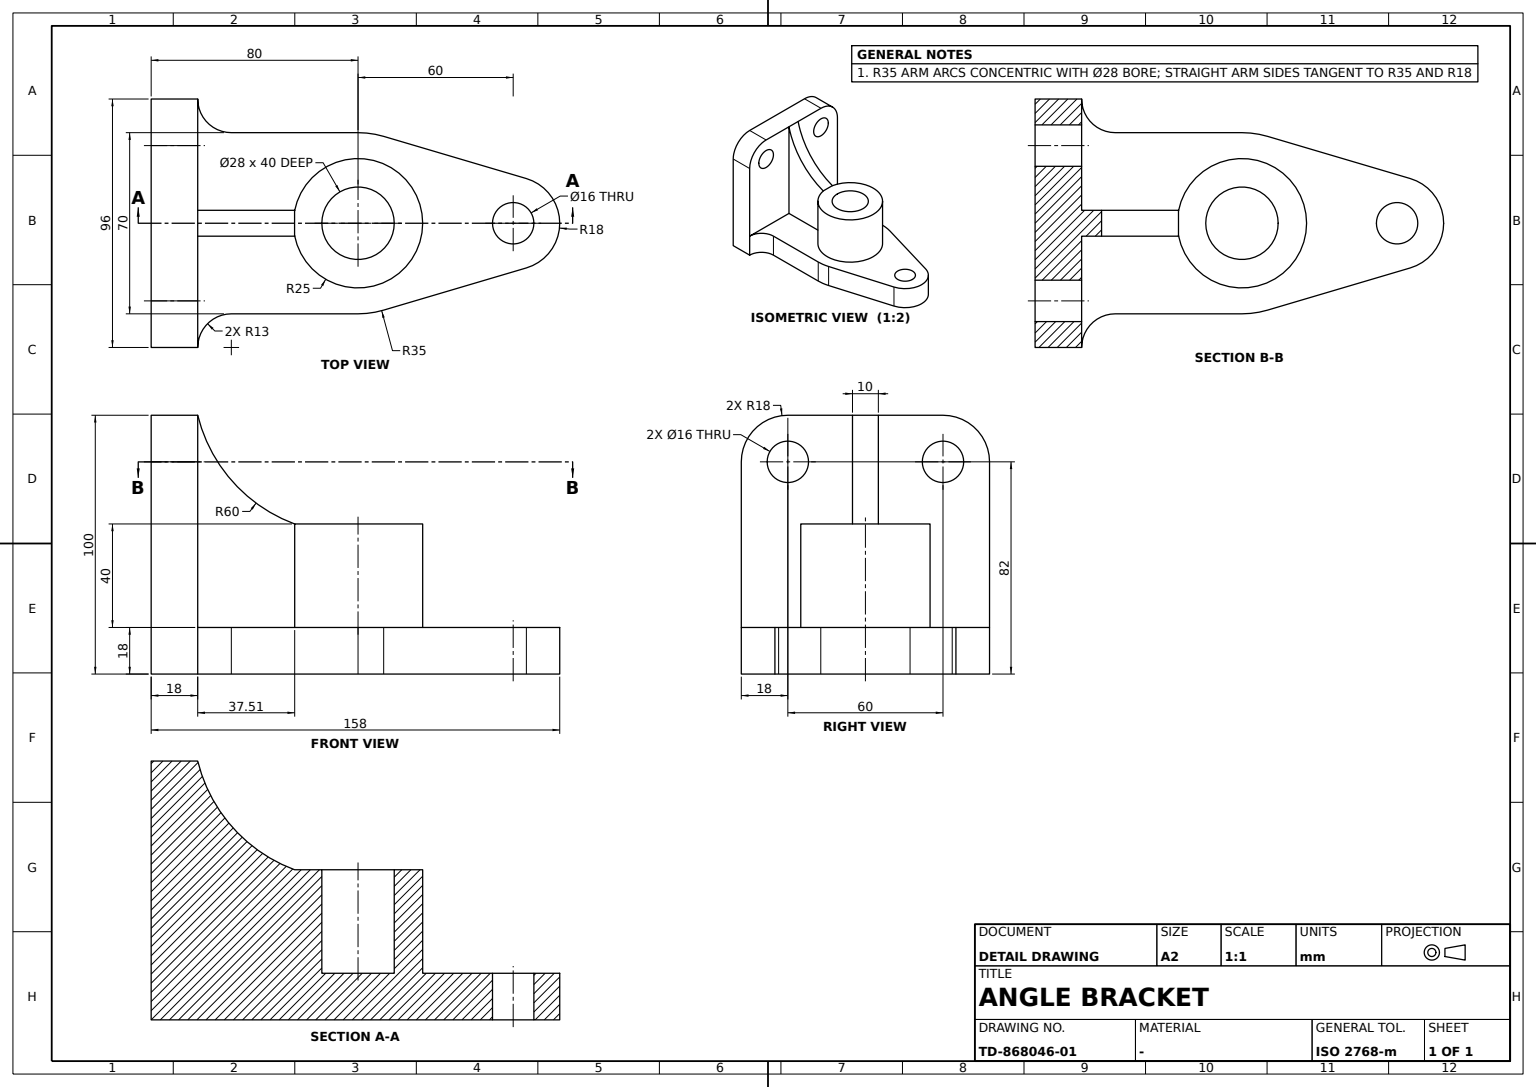
ISO-10303-21;
HEADER;
FILE_DESCRIPTION((''),'2;1');
FILE_NAME('','',(''),(''),'','','');
FILE_SCHEMA(('AUTOMOTIVE_DESIGN'));
ENDSEC;
DATA;
#1=APPLICATION_CONTEXT('');
#2=PRODUCT_CONTEXT('',#1,'mechanical');
#3=PRODUCT('','','',(#2));
#4=PRODUCT_DEFINITION_FORMATION('','',#3);
#5=PRODUCT_DEFINITION_CONTEXT('',#1,'design');
#6=PRODUCT_DEFINITION('','',#4,#5);
#7=PRODUCT_DEFINITION_SHAPE('','',#6);
#8=(LENGTH_UNIT()NAMED_UNIT(*)SI_UNIT(.MILLI.,.METRE.));
#9=(NAMED_UNIT(*)PLANE_ANGLE_UNIT()SI_UNIT($,.RADIAN.));
#10=(NAMED_UNIT(*)SI_UNIT($,.STERADIAN.)SOLID_ANGLE_UNIT());
#11=UNCERTAINTY_MEASURE_WITH_UNIT(LENGTH_MEASURE(1.E-05),#8,'distance_accuracy_value','');
#12=(GEOMETRIC_REPRESENTATION_CONTEXT(3)GLOBAL_UNCERTAINTY_ASSIGNED_CONTEXT((#11))GLOBAL_UNIT_ASSIGNED_CONTEXT((#8,#9,#10))REPRESENTATION_CONTEXT('',''));
#13=CARTESIAN_POINT('',(18.,5.,18.));
#14=VERTEX_POINT('',#13);
#15=CARTESIAN_POINT('',(55.505103,5.,18.));
#16=VERTEX_POINT('',#15);
#17=CARTESIAN_POINT('',(36.752551,5.,18.));
#18=DIRECTION('',(1.,0.,0.));
#19=VECTOR('',#18,1000.);
#20=LINE('',#17,#19);
#21=EDGE_CURVE('',#14,#16,#20,.T.);
#22=ORIENTED_EDGE('',*,*,#21,.F.);
#23=CARTESIAN_POINT('',(18.,5.,100.));
#24=VERTEX_POINT('',#23);
#25=CARTESIAN_POINT('',(18.,5.,59.));
#26=DIRECTION('',(0.,0.,-1.));
#27=VECTOR('',#26,1000.);
#28=LINE('',#25,#27);
#29=EDGE_CURVE('',#24,#14,#28,.T.);
#30=ORIENTED_EDGE('',*,*,#29,.F.);
#31=CARTESIAN_POINT('',(55.458542,5.,58.));
#32=VERTEX_POINT('',#31);
#33=CARTESIAN_POINT('',(76.277827,5.,114.272172));
#34=DIRECTION('',(0.,1.,0.));
#35=DIRECTION('',(-1.,0.,0.));
#36=AXIS2_PLACEMENT_3D('',#33,#34,#35);
#37=CIRCLE('',#36,60.);
#38=EDGE_CURVE('',#32,#24,#37,.T.);
#39=ORIENTED_EDGE('',*,*,#38,.F.);
#40=CARTESIAN_POINT('',(55.505103,5.,57.982774));
#41=VERTEX_POINT('',#40);
#42=CARTESIAN_POINT('',(55.481822,5.,57.991387));
#43=DIRECTION('',(-0.937869538,0.,0.346988082));
#44=VECTOR('',#43,1000.);
#45=LINE('',#42,#44);
#46=EDGE_CURVE('',#41,#32,#45,.T.);
#47=ORIENTED_EDGE('',*,*,#46,.F.);
#48=CARTESIAN_POINT('',(55.505103,5.,37.991387));
#49=DIRECTION('',(0.,0.,1.));
#50=VECTOR('',#49,1000.);
#51=LINE('',#48,#50);
#52=EDGE_CURVE('',#16,#41,#51,.T.);
#53=ORIENTED_EDGE('',*,*,#52,.F.);
#54=EDGE_LOOP('',(#22,#30,#39,#47,#53));
#55=FACE_OUTER_BOUND('',#54,.T.);
#56=CARTESIAN_POINT('',(0.,5.,0.));
#57=AXIS2_PLACEMENT_3D('',#56,#34,#35);
#58=PLANE('',#57);
#59=ADVANCED_FACE('',(#55),#58,.T.);
#60=CARTESIAN_POINT('',(18.,48.,18.));
#61=VERTEX_POINT('',#60);
#62=CARTESIAN_POINT('',(18.,26.5,18.));
#63=VECTOR('',#34,1000.);
#64=LINE('',#62,#63);
#65=EDGE_CURVE('',#14,#61,#64,.T.);
#66=ORIENTED_EDGE('',*,*,#65,.T.);
#67=CARTESIAN_POINT('',(18.,48.,82.));
#68=VERTEX_POINT('',#67);
#69=CARTESIAN_POINT('',(18.,48.,50.));
#70=LINE('',#69,#27);
#71=EDGE_CURVE('',#68,#61,#70,.T.);
#72=ORIENTED_EDGE('',*,*,#71,.F.);
#73=CARTESIAN_POINT('',(18.,30.,100.));
#74=VERTEX_POINT('',#73);
#75=CARTESIAN_POINT('',(18.,30.,82.));
#76=AXIS2_PLACEMENT_3D('',#75,#35,#26);
#77=CIRCLE('',#76,18.);
#78=EDGE_CURVE('',#74,#68,#77,.T.);
#79=ORIENTED_EDGE('',*,*,#78,.F.);
#80=CARTESIAN_POINT('',(18.,17.5,100.));
#81=LINE('',#80,#63);
#82=EDGE_CURVE('',#24,#74,#81,.T.);
#83=ORIENTED_EDGE('',*,*,#82,.F.);
#84=ORIENTED_EDGE('',*,*,#29,.T.);
#85=EDGE_LOOP('',(#66,#72,#79,#83,#84));
#86=FACE_OUTER_BOUND('',#85,.T.);
#87=CARTESIAN_POINT('',(18.,22.,82.));
#88=VERTEX_POINT('',#87);
#89=CARTESIAN_POINT('',(18.,38.,82.));
#90=VERTEX_POINT('',#89);
#91=AXIS2_PLACEMENT_3D('',#75,#18,#34);
#92=CIRCLE('',#91,8.);
#93=EDGE_CURVE('',#88,#90,#92,.T.);
#94=ORIENTED_EDGE('',*,*,#93,.F.);
#95=EDGE_CURVE('',#90,#88,#92,.T.);
#96=ORIENTED_EDGE('',*,*,#95,.F.);
#97=EDGE_LOOP('',(#94,#96));
#98=FACE_BOUND('',#97,.T.);
#99=CARTESIAN_POINT('',(18.,0.,100.));
#100=AXIS2_PLACEMENT_3D('',#99,#18,#26);
#101=PLANE('',#100);
#102=ADVANCED_FACE('',(#86,#98),#101,.T.);
#103=CARTESIAN_POINT('',(0.,-22.,82.));
#104=VERTEX_POINT('',#103);
#105=CARTESIAN_POINT('',(0.,-38.,82.));
#106=VERTEX_POINT('',#105);
#107=CARTESIAN_POINT('',(0.,-30.,82.));
#108=AXIS2_PLACEMENT_3D('',#107,#35,#49);
#109=CIRCLE('',#108,8.);
#110=EDGE_CURVE('',#104,#106,#109,.T.);
#111=ORIENTED_EDGE('',*,*,#110,.T.);
#112=CARTESIAN_POINT('',(18.,-38.,82.));
#113=VERTEX_POINT('',#112);
#114=CARTESIAN_POINT('',(-6.,-38.,82.));
#115=VECTOR('',#35,1000.);
#116=LINE('',#114,#115);
#117=EDGE_CURVE('',#113,#106,#116,.T.);
#118=ORIENTED_EDGE('',*,*,#117,.F.);
#119=CARTESIAN_POINT('',(18.,-22.,82.));
#120=VERTEX_POINT('',#119);
#121=CARTESIAN_POINT('',(18.,-30.,82.));
#122=AXIS2_PLACEMENT_3D('',#121,#18,#34);
#123=CIRCLE('',#122,8.);
#124=EDGE_CURVE('',#113,#120,#123,.T.);
#125=ORIENTED_EDGE('',*,*,#124,.T.);
#126=CARTESIAN_POINT('',(-6.,-22.,82.));
#127=LINE('',#126,#115);
#128=EDGE_CURVE('',#120,#104,#127,.T.);
#129=ORIENTED_EDGE('',*,*,#128,.T.);
#130=EDGE_LOOP('',(#111,#118,#125,#129));
#131=FACE_OUTER_BOUND('',#130,.T.);
#132=CARTESIAN_POINT('',(-6.,-30.,82.));
#133=AXIS2_PLACEMENT_3D('',#132,#35,#34);
#134=CYLINDRICAL_SURFACE('',#133,8.);
#135=ADVANCED_FACE('',(#131),#134,.F.);
#136=CARTESIAN_POINT('',(0.,22.,82.));
#137=VERTEX_POINT('',#136);
#138=CARTESIAN_POINT('',(-6.,22.,82.));
#139=LINE('',#138,#115);
#140=EDGE_CURVE('',#88,#137,#139,.T.);
#141=ORIENTED_EDGE('',*,*,#140,.T.);
#142=CARTESIAN_POINT('',(0.,38.,82.));
#143=VERTEX_POINT('',#142);
#144=CARTESIAN_POINT('',(0.,30.,82.));
#145=AXIS2_PLACEMENT_3D('',#144,#35,#49);
#146=CIRCLE('',#145,8.);
#147=EDGE_CURVE('',#137,#143,#146,.T.);
#148=ORIENTED_EDGE('',*,*,#147,.T.);
#149=CARTESIAN_POINT('',(-6.,38.,82.));
#150=LINE('',#149,#115);
#151=EDGE_CURVE('',#90,#143,#150,.T.);
#152=ORIENTED_EDGE('',*,*,#151,.F.);
#153=ORIENTED_EDGE('',*,*,#95,.T.);
#154=EDGE_LOOP('',(#141,#148,#152,#153));
#155=FACE_OUTER_BOUND('',#154,.T.);
#156=CARTESIAN_POINT('',(-6.,30.,82.));
#157=AXIS2_PLACEMENT_3D('',#156,#35,#34);
#158=CYLINDRICAL_SURFACE('',#157,8.);
#159=ADVANCED_FACE('',(#155),#158,.F.);
#160=ORIENTED_EDGE('',*,*,#110,.F.);
#161=EDGE_CURVE('',#106,#104,#109,.T.);
#162=ORIENTED_EDGE('',*,*,#161,.F.);
#163=EDGE_LOOP('',(#160,#162));
#164=FACE_BOUND('',#163,.T.);
#165=CARTESIAN_POINT('',(0.,-30.,100.));
#166=VERTEX_POINT('',#165);
#167=CARTESIAN_POINT('',(0.,30.,100.));
#168=VERTEX_POINT('',#167);
#169=CARTESIAN_POINT('',(0.,0.,100.));
#170=LINE('',#169,#63);
#171=EDGE_CURVE('',#166,#168,#170,.T.);
#172=ORIENTED_EDGE('',*,*,#171,.T.);
#173=CARTESIAN_POINT('',(0.,48.,82.));
#174=VERTEX_POINT('',#173);
#175=AXIS2_PLACEMENT_3D('',#144,#18,#49);
#176=CIRCLE('',#175,18.);
#177=EDGE_CURVE('',#174,#168,#176,.T.);
#178=ORIENTED_EDGE('',*,*,#177,.F.);
#179=CARTESIAN_POINT('',(0.,48.,0.));
#180=VERTEX_POINT('',#179);
#181=CARTESIAN_POINT('',(0.,48.,41.));
#182=LINE('',#181,#50);
#183=EDGE_CURVE('',#180,#174,#182,.T.);
#184=ORIENTED_EDGE('',*,*,#183,.F.);
#185=CARTESIAN_POINT('',(0.,-48.,0.));
#186=VERTEX_POINT('',#185);
#187=CARTESIAN_POINT('',(0.,0.,0.));
#188=LINE('',#187,#63);
#189=EDGE_CURVE('',#186,#180,#188,.T.);
#190=ORIENTED_EDGE('',*,*,#189,.F.);
#191=CARTESIAN_POINT('',(0.,-48.,82.));
#192=VERTEX_POINT('',#191);
#193=CARTESIAN_POINT('',(0.,-48.,41.));
#194=LINE('',#193,#50);
#195=EDGE_CURVE('',#186,#192,#194,.T.);
#196=ORIENTED_EDGE('',*,*,#195,.T.);
#197=AXIS2_PLACEMENT_3D('',#107,#18,#49);
#198=CIRCLE('',#197,18.);
#199=EDGE_CURVE('',#166,#192,#198,.T.);
#200=ORIENTED_EDGE('',*,*,#199,.F.);
#201=EDGE_LOOP('',(#172,#178,#184,#190,#196,#200));
#202=FACE_OUTER_BOUND('',#201,.T.);
#203=EDGE_CURVE('',#143,#137,#146,.T.);
#204=ORIENTED_EDGE('',*,*,#203,.F.);
#205=ORIENTED_EDGE('',*,*,#147,.F.);
#206=EDGE_LOOP('',(#204,#205));
#207=FACE_BOUND('',#206,.T.);
#208=AXIS2_PLACEMENT_3D('',#187,#35,#49);
#209=PLANE('',#208);
#210=ADVANCED_FACE('',(#164,#202,#207),#209,.T.);
#211=ORIENTED_EDGE('',*,*,#195,.F.);
#212=CARTESIAN_POINT('',(18.,-48.,0.));
#213=VERTEX_POINT('',#212);
#214=CARTESIAN_POINT('',(9.,-48.,0.));
#215=LINE('',#214,#115);
#216=EDGE_CURVE('',#213,#186,#215,.T.);
#217=ORIENTED_EDGE('',*,*,#216,.F.);
#218=CARTESIAN_POINT('',(18.,-48.,18.));
#219=VERTEX_POINT('',#218);
#220=CARTESIAN_POINT('',(18.,-48.,9.));
#221=LINE('',#220,#50);
#222=EDGE_CURVE('',#213,#219,#221,.T.);
#223=ORIENTED_EDGE('',*,*,#222,.T.);
#224=CARTESIAN_POINT('',(18.,-48.,82.));
#225=VERTEX_POINT('',#224);
#226=CARTESIAN_POINT('',(18.,-48.,50.));
#227=LINE('',#226,#27);
#228=EDGE_CURVE('',#225,#219,#227,.T.);
#229=ORIENTED_EDGE('',*,*,#228,.F.);
#230=CARTESIAN_POINT('',(9.,-48.,82.));
#231=LINE('',#230,#19);
#232=EDGE_CURVE('',#192,#225,#231,.T.);
#233=ORIENTED_EDGE('',*,*,#232,.F.);
#234=EDGE_LOOP('',(#211,#217,#223,#229,#233));
#235=FACE_OUTER_BOUND('',#234,.T.);
#236=AXIS2_PLACEMENT_3D('',#185,#34,#35);
#237=PLANE('',#236);
#238=ADVANCED_FACE('',(#235),#237,.F.);
#239=EDGE_CURVE('',#120,#113,#123,.T.);
#240=ORIENTED_EDGE('',*,*,#239,.F.);
#241=ORIENTED_EDGE('',*,*,#124,.F.);
#242=EDGE_LOOP('',(#240,#241));
#243=FACE_BOUND('',#242,.T.);
#244=CARTESIAN_POINT('',(18.,-5.,100.));
#245=VERTEX_POINT('',#244);
#246=CARTESIAN_POINT('',(18.,-5.,18.));
#247=VERTEX_POINT('',#246);
#248=CARTESIAN_POINT('',(18.,-5.,59.));
#249=LINE('',#248,#27);
#250=EDGE_CURVE('',#245,#247,#249,.T.);
#251=ORIENTED_EDGE('',*,*,#250,.F.);
#252=CARTESIAN_POINT('',(18.,-30.,100.));
#253=VERTEX_POINT('',#252);
#254=CARTESIAN_POINT('',(18.,-17.5,100.));
#255=LINE('',#254,#63);
#256=EDGE_CURVE('',#253,#245,#255,.T.);
#257=ORIENTED_EDGE('',*,*,#256,.F.);
#258=AXIS2_PLACEMENT_3D('',#121,#35,#26);
#259=CIRCLE('',#258,18.);
#260=EDGE_CURVE('',#225,#253,#259,.T.);
#261=ORIENTED_EDGE('',*,*,#260,.F.);
#262=ORIENTED_EDGE('',*,*,#228,.T.);
#263=CARTESIAN_POINT('',(18.,-26.5,18.));
#264=LINE('',#263,#63);
#265=EDGE_CURVE('',#219,#247,#264,.T.);
#266=ORIENTED_EDGE('',*,*,#265,.T.);
#267=EDGE_LOOP('',(#251,#257,#261,#262,#266));
#268=FACE_OUTER_BOUND('',#267,.T.);
#269=ADVANCED_FACE('',(#243,#268),#101,.T.);
#270=CARTESIAN_POINT('',(66.,0.,58.));
#271=VERTEX_POINT('',#270);
#272=CARTESIAN_POINT('',(94.,0.,58.));
#273=VERTEX_POINT('',#272);
#274=CARTESIAN_POINT('',(80.,0.,58.));
#275=AXIS2_PLACEMENT_3D('',#274,#49,#18);
#276=CIRCLE('',#275,14.);
#277=EDGE_CURVE('',#271,#273,#276,.T.);
#278=ORIENTED_EDGE('',*,*,#277,.F.);
#279=EDGE_CURVE('',#273,#271,#276,.T.);
#280=ORIENTED_EDGE('',*,*,#279,.F.);
#281=EDGE_LOOP('',(#278,#280));
#282=FACE_BOUND('',#281,.T.);
#283=CARTESIAN_POINT('',(55.458542,-4.766218,58.));
#284=VERTEX_POINT('',#283);
#285=CARTESIAN_POINT('',(105.,0.,58.));
#286=VERTEX_POINT('',#285);
#287=CIRCLE('',#275,25.);
#288=EDGE_CURVE('',#284,#286,#287,.T.);
#289=ORIENTED_EDGE('',*,*,#288,.T.);
#290=CARTESIAN_POINT('',(55.458542,4.766218,58.));
#291=VERTEX_POINT('',#290);
#292=EDGE_CURVE('',#286,#291,#287,.T.);
#293=ORIENTED_EDGE('',*,*,#292,.T.);
#294=CARTESIAN_POINT('',(55.458542,0.,58.));
#295=LINE('',#294,#63);
#296=EDGE_CURVE('',#284,#291,#295,.T.);
#297=ORIENTED_EDGE('',*,*,#296,.F.);
#298=EDGE_LOOP('',(#289,#293,#297));
#299=FACE_OUTER_BOUND('',#298,.T.);
#300=CARTESIAN_POINT('',(0.,0.,58.));
#301=AXIS2_PLACEMENT_3D('',#300,#49,#18);
#302=PLANE('',#301);
#303=ADVANCED_FACE('',(#282,#299),#302,.T.);
#304=CARTESIAN_POINT('',(55.467632,4.813024,57.996637));
#305=CARTESIAN_POINT('',(55.476833,4.859806,57.993233));
#306=CARTESIAN_POINT('',(55.486146,4.906563,57.989787));
#307=CARTESIAN_POINT('',(55.495569,4.953294,57.986301));
#308=B_SPLINE_CURVE_WITH_KNOTS('',5,(#290,#304,#305,#306,#307,#40),.UNSPECIFIED.,.F.,.F.,(6,6),(0.,0.337990946),.UNSPECIFIED.);
#309=EDGE_CURVE('',#291,#41,#308,.T.);
#310=ORIENTED_EDGE('',*,*,#309,.T.);
#311=ORIENTED_EDGE('',*,*,#46,.T.);
#312=CARTESIAN_POINT('',(55.458542,4.883109,58.));
#313=LINE('',#312,#63);
#314=EDGE_CURVE('',#291,#32,#313,.T.);
#315=ORIENTED_EDGE('',*,*,#314,.F.);
#316=EDGE_LOOP('',(#310,#311,#315));
#317=FACE_OUTER_BOUND('',#316,.T.);
#318=DIRECTION('',(0.346988082,0.,0.937869538));
#319=DIRECTION('',(0.937869538,0.,-0.346988082));
#320=AXIS2_PLACEMENT_3D('',#294,#318,#319);
#321=PLANE('',#320);
#322=ADVANCED_FACE('',(#317),#321,.T.);
#323=CARTESIAN_POINT('',(9.,-30.,100.));
#324=LINE('',#323,#19);
#325=EDGE_CURVE('',#166,#253,#324,.T.);
#326=ORIENTED_EDGE('',*,*,#325,.F.);
#327=ORIENTED_EDGE('',*,*,#199,.T.);
#328=ORIENTED_EDGE('',*,*,#232,.T.);
#329=ORIENTED_EDGE('',*,*,#260,.T.);
#330=EDGE_LOOP('',(#326,#327,#328,#329));
#331=FACE_OUTER_BOUND('',#330,.T.);
#332=CARTESIAN_POINT('',(9.,-30.,82.));
#333=DIRECTION('',(0.,-1.,0.));
#334=AXIS2_PLACEMENT_3D('',#332,#35,#333);
#335=CYLINDRICAL_SURFACE('',#334,18.);
#336=ADVANCED_FACE('',(#331),#335,.T.);
#337=CARTESIAN_POINT('',(105.,0.,18.));
#338=VERTEX_POINT('',#337);
#339=CARTESIAN_POINT('',(105.,0.,38.));
#340=LINE('',#339,#50);
#341=EDGE_CURVE('',#338,#286,#340,.T.);
#342=ORIENTED_EDGE('',*,*,#341,.T.);
#343=ORIENTED_EDGE('',*,*,#288,.F.);
#344=CARTESIAN_POINT('',(55.505103,-5.,57.982774));
#345=VERTEX_POINT('',#344);
#346=CARTESIAN_POINT('',(55.467632,-4.813024,57.996637));
#347=CARTESIAN_POINT('',(55.476833,-4.859806,57.993233));
#348=CARTESIAN_POINT('',(55.486146,-4.906563,57.989787));
#349=CARTESIAN_POINT('',(55.495569,-4.953294,57.986301));
#350=B_SPLINE_CURVE_WITH_KNOTS('',5,(#283,#346,#347,#348,#349,#344),.UNSPECIFIED.,.F.,.F.,(6,6),(0.,0.337990946),.UNSPECIFIED.);
#351=EDGE_CURVE('',#284,#345,#350,.T.);
#352=ORIENTED_EDGE('',*,*,#351,.T.);
#353=CARTESIAN_POINT('',(55.505103,-5.,18.));
#354=VERTEX_POINT('',#353);
#355=CARTESIAN_POINT('',(55.505103,-5.,37.991387));
#356=LINE('',#355,#50);
#357=EDGE_CURVE('',#354,#345,#356,.T.);
#358=ORIENTED_EDGE('',*,*,#357,.F.);
#359=CARTESIAN_POINT('',(80.,0.,18.));
#360=AXIS2_PLACEMENT_3D('',#359,#49,#18);
#361=CIRCLE('',#360,25.);
#362=EDGE_CURVE('',#354,#338,#361,.T.);
#363=ORIENTED_EDGE('',*,*,#362,.T.);
#364=EDGE_LOOP('',(#342,#343,#352,#358,#363));
#365=FACE_OUTER_BOUND('',#364,.T.);
#366=CARTESIAN_POINT('',(80.,0.,38.));
#367=AXIS2_PLACEMENT_3D('',#366,#26,#18);
#368=CYLINDRICAL_SURFACE('',#367,25.);
#369=ADVANCED_FACE('',(#365),#368,.T.);
#370=CARTESIAN_POINT('',(158.,0.,18.));
#371=VERTEX_POINT('',#370);
#372=CARTESIAN_POINT('',(158.,0.,0.));
#373=VERTEX_POINT('',#372);
#374=CARTESIAN_POINT('',(158.,0.,9.));
#375=LINE('',#374,#27);
#376=EDGE_CURVE('',#371,#373,#375,.T.);
#377=ORIENTED_EDGE('',*,*,#376,.F.);
#378=CARTESIAN_POINT('',(145.1,-17.262387,18.));
#379=VERTEX_POINT('',#378);
#380=CARTESIAN_POINT('',(140.,0.,18.));
#381=AXIS2_PLACEMENT_3D('',#380,#49,#18);
#382=CIRCLE('',#381,18.);
#383=EDGE_CURVE('',#379,#371,#382,.T.);
#384=ORIENTED_EDGE('',*,*,#383,.F.);
#385=CARTESIAN_POINT('',(145.1,-17.262387,0.));
#386=VERTEX_POINT('',#385);
#387=CARTESIAN_POINT('',(145.1,-17.262387,9.));
#388=LINE('',#387,#50);
#389=EDGE_CURVE('',#386,#379,#388,.T.);
#390=ORIENTED_EDGE('',*,*,#389,.F.);
#391=CARTESIAN_POINT('',(140.,0.,0.));
#392=AXIS2_PLACEMENT_3D('',#391,#49,#18);
#393=CIRCLE('',#392,18.);
#394=EDGE_CURVE('',#386,#373,#393,.T.);
#395=ORIENTED_EDGE('',*,*,#394,.T.);
#396=EDGE_LOOP('',(#377,#384,#390,#395));
#397=FACE_OUTER_BOUND('',#396,.T.);
#398=CARTESIAN_POINT('',(140.,0.,9.));
#399=AXIS2_PLACEMENT_3D('',#398,#26,#18);
#400=CYLINDRICAL_SURFACE('',#399,18.);
#401=ADVANCED_FACE('',(#397),#400,.T.);
#402=CARTESIAN_POINT('',(80.,-35.,0.));
#403=VERTEX_POINT('',#402);
#404=CARTESIAN_POINT('',(80.,-35.,18.));
#405=VERTEX_POINT('',#404);
#406=CARTESIAN_POINT('',(80.,-35.,9.));
#407=LINE('',#406,#50);
#408=EDGE_CURVE('',#403,#405,#407,.T.);
#409=ORIENTED_EDGE('',*,*,#408,.F.);
#410=CARTESIAN_POINT('',(89.916667,-33.565752,0.));
#411=VERTEX_POINT('',#410);
#412=CARTESIAN_POINT('',(80.,0.,0.));
#413=AXIS2_PLACEMENT_3D('',#412,#49,#18);
#414=CIRCLE('',#413,35.);
#415=EDGE_CURVE('',#403,#411,#414,.T.);
#416=ORIENTED_EDGE('',*,*,#415,.T.);
#417=CARTESIAN_POINT('',(89.916667,-33.565752,18.));
#418=VERTEX_POINT('',#417);
#419=CARTESIAN_POINT('',(89.916667,-33.565752,9.));
#420=LINE('',#419,#50);
#421=EDGE_CURVE('',#411,#418,#420,.T.);
#422=ORIENTED_EDGE('',*,*,#421,.T.);
#423=CIRCLE('',#360,35.);
#424=EDGE_CURVE('',#405,#418,#423,.T.);
#425=ORIENTED_EDGE('',*,*,#424,.F.);
#426=EDGE_LOOP('',(#409,#416,#422,#425));
#427=FACE_OUTER_BOUND('',#426,.T.);
#428=CARTESIAN_POINT('',(80.,0.,9.));
#429=AXIS2_PLACEMENT_3D('',#428,#26,#18);
#430=CYLINDRICAL_SURFACE('',#429,35.);
#431=ADVANCED_FACE('',(#427),#430,.T.);
#432=CARTESIAN_POINT('',(148.,0.,0.));
#433=VERTEX_POINT('',#432);
#434=CARTESIAN_POINT('',(132.,0.,0.));
#435=VERTEX_POINT('',#434);
#436=AXIS2_PLACEMENT_3D('',#391,#26,#35);
#437=CIRCLE('',#436,8.);
#438=EDGE_CURVE('',#433,#435,#437,.T.);
#439=ORIENTED_EDGE('',*,*,#438,.F.);
#440=EDGE_CURVE('',#435,#433,#437,.T.);
#441=ORIENTED_EDGE('',*,*,#440,.F.);
#442=EDGE_LOOP('',(#439,#441));
#443=FACE_BOUND('',#442,.T.);
#444=ORIENTED_EDGE('',*,*,#216,.T.);
#445=ORIENTED_EDGE('',*,*,#189,.T.);
#446=CARTESIAN_POINT('',(18.,48.,0.));
#447=VERTEX_POINT('',#446);
#448=CARTESIAN_POINT('',(9.,48.,0.));
#449=LINE('',#448,#115);
#450=EDGE_CURVE('',#447,#180,#449,.T.);
#451=ORIENTED_EDGE('',*,*,#450,.F.);
#452=CARTESIAN_POINT('',(31.,35.,0.));
#453=VERTEX_POINT('',#452);
#454=CARTESIAN_POINT('',(31.,48.,0.));
#455=AXIS2_PLACEMENT_3D('',#454,#49,#35);
#456=CIRCLE('',#455,13.);
#457=EDGE_CURVE('',#447,#453,#456,.T.);
#458=ORIENTED_EDGE('',*,*,#457,.T.);
#459=CARTESIAN_POINT('',(80.,35.,0.));
#460=VERTEX_POINT('',#459);
#461=CARTESIAN_POINT('',(55.5,35.,0.));
#462=LINE('',#461,#115);
#463=EDGE_CURVE('',#460,#453,#462,.T.);
#464=ORIENTED_EDGE('',*,*,#463,.F.);
#465=CARTESIAN_POINT('',(89.916667,33.565752,0.));
#466=VERTEX_POINT('',#465);
#467=EDGE_CURVE('',#466,#460,#414,.T.);
#468=ORIENTED_EDGE('',*,*,#467,.F.);
#469=CARTESIAN_POINT('',(145.1,17.262387,0.));
#470=VERTEX_POINT('',#469);
#471=CARTESIAN_POINT('',(117.508333,25.41407,0.));
#472=DIRECTION('',(-0.959021492,0.283333333,0.));
#473=VECTOR('',#472,1000.);
#474=LINE('',#471,#473);
#475=EDGE_CURVE('',#470,#466,#474,.T.);
#476=ORIENTED_EDGE('',*,*,#475,.F.);
#477=EDGE_CURVE('',#373,#470,#393,.T.);
#478=ORIENTED_EDGE('',*,*,#477,.F.);
#479=ORIENTED_EDGE('',*,*,#394,.F.);
#480=CARTESIAN_POINT('',(117.508333,-25.41407,0.));
#481=DIRECTION('',(0.959021492,0.283333333,0.));
#482=VECTOR('',#481,1000.);
#483=LINE('',#480,#482);
#484=EDGE_CURVE('',#411,#386,#483,.T.);
#485=ORIENTED_EDGE('',*,*,#484,.F.);
#486=ORIENTED_EDGE('',*,*,#415,.F.);
#487=CARTESIAN_POINT('',(31.,-35.,0.));
#488=VERTEX_POINT('',#487);
#489=CARTESIAN_POINT('',(55.5,-35.,0.));
#490=LINE('',#489,#19);
#491=EDGE_CURVE('',#488,#403,#490,.T.);
#492=ORIENTED_EDGE('',*,*,#491,.F.);
#493=CARTESIAN_POINT('',(31.,-48.,0.));
#494=AXIS2_PLACEMENT_3D('',#493,#49,#35);
#495=CIRCLE('',#494,13.);
#496=EDGE_CURVE('',#488,#213,#495,.T.);
#497=ORIENTED_EDGE('',*,*,#496,.T.);
#498=EDGE_LOOP('',(#444,#445,#451,#458,#464,#468,#476,#478,#479,#485,#486,#492,#497));
#499=FACE_OUTER_BOUND('',#498,.T.);
#500=CARTESIAN_POINT('',(18.,0.,0.));
#501=AXIS2_PLACEMENT_3D('',#500,#26,#35);
#502=PLANE('',#501);
#503=ADVANCED_FACE('',(#443,#499),#502,.T.);
#504=ORIENTED_EDGE('',*,*,#484,.T.);
#505=ORIENTED_EDGE('',*,*,#389,.T.);
#506=CARTESIAN_POINT('',(117.508333,-25.41407,18.));
#507=LINE('',#506,#482);
#508=EDGE_CURVE('',#418,#379,#507,.T.);
#509=ORIENTED_EDGE('',*,*,#508,.F.);
#510=ORIENTED_EDGE('',*,*,#421,.F.);
#511=EDGE_LOOP('',(#504,#505,#509,#510));
#512=FACE_OUTER_BOUND('',#511,.T.);
#513=DIRECTION('',(0.283333333,-0.959021492,0.));
#514=AXIS2_PLACEMENT_3D('',#410,#513,#481);
#515=PLANE('',#514);
#516=ADVANCED_FACE('',(#512),#515,.T.);
#517=EDGE_CURVE('',#338,#16,#361,.T.);
#518=ORIENTED_EDGE('',*,*,#517,.T.);
#519=ORIENTED_EDGE('',*,*,#52,.T.);
#520=ORIENTED_EDGE('',*,*,#309,.F.);
#521=ORIENTED_EDGE('',*,*,#292,.F.);
#522=ORIENTED_EDGE('',*,*,#341,.F.);
#523=EDGE_LOOP('',(#518,#519,#520,#521,#522));
#524=FACE_OUTER_BOUND('',#523,.T.);
#525=ADVANCED_FACE('',(#524),#368,.T.);
#526=ORIENTED_EDGE('',*,*,#140,.F.);
#527=ORIENTED_EDGE('',*,*,#93,.T.);
#528=ORIENTED_EDGE('',*,*,#151,.T.);
#529=ORIENTED_EDGE('',*,*,#203,.T.);
#530=EDGE_LOOP('',(#526,#527,#528,#529));
#531=FACE_OUTER_BOUND('',#530,.T.);
#532=ADVANCED_FACE('',(#531),#158,.F.);
#533=CARTESIAN_POINT('',(31.,-35.,18.));
#534=VERTEX_POINT('',#533);
#535=CARTESIAN_POINT('',(31.,-48.,18.));
#536=AXIS2_PLACEMENT_3D('',#535,#26,#18);
#537=CIRCLE('',#536,13.);
#538=EDGE_CURVE('',#219,#534,#537,.T.);
#539=ORIENTED_EDGE('',*,*,#538,.F.);
#540=ORIENTED_EDGE('',*,*,#222,.F.);
#541=ORIENTED_EDGE('',*,*,#496,.F.);
#542=CARTESIAN_POINT('',(31.,-35.,9.));
#543=LINE('',#542,#50);
#544=EDGE_CURVE('',#488,#534,#543,.T.);
#545=ORIENTED_EDGE('',*,*,#544,.T.);
#546=EDGE_LOOP('',(#539,#540,#541,#545));
#547=FACE_OUTER_BOUND('',#546,.T.);
#548=CARTESIAN_POINT('',(31.,-48.,50.));
#549=AXIS2_PLACEMENT_3D('',#548,#26,#35);
#550=CYLINDRICAL_SURFACE('',#549,13.);
#551=ADVANCED_FACE('',(#547),#550,.F.);
#552=ORIENTED_EDGE('',*,*,#517,.F.);
#553=ORIENTED_EDGE('',*,*,#362,.F.);
#554=CARTESIAN_POINT('',(36.752551,-5.,18.));
#555=LINE('',#554,#19);
#556=EDGE_CURVE('',#247,#354,#555,.T.);
#557=ORIENTED_EDGE('',*,*,#556,.F.);
#558=ORIENTED_EDGE('',*,*,#265,.F.);
#559=ORIENTED_EDGE('',*,*,#538,.T.);
#560=CARTESIAN_POINT('',(55.5,-35.,18.));
#561=LINE('',#560,#19);
#562=EDGE_CURVE('',#534,#405,#561,.T.);
#563=ORIENTED_EDGE('',*,*,#562,.T.);
#564=ORIENTED_EDGE('',*,*,#424,.T.);
#565=ORIENTED_EDGE('',*,*,#508,.T.);
#566=ORIENTED_EDGE('',*,*,#383,.T.);
#567=CARTESIAN_POINT('',(145.1,17.262387,18.));
#568=VERTEX_POINT('',#567);
#569=EDGE_CURVE('',#371,#568,#382,.T.);
#570=ORIENTED_EDGE('',*,*,#569,.T.);
#571=CARTESIAN_POINT('',(89.916667,33.565752,18.));
#572=VERTEX_POINT('',#571);
#573=CARTESIAN_POINT('',(117.508333,25.41407,18.));
#574=LINE('',#573,#473);
#575=EDGE_CURVE('',#568,#572,#574,.T.);
#576=ORIENTED_EDGE('',*,*,#575,.T.);
#577=CARTESIAN_POINT('',(80.,35.,18.));
#578=VERTEX_POINT('',#577);
#579=EDGE_CURVE('',#572,#578,#423,.T.);
#580=ORIENTED_EDGE('',*,*,#579,.T.);
#581=CARTESIAN_POINT('',(31.,35.,18.));
#582=VERTEX_POINT('',#581);
#583=CARTESIAN_POINT('',(55.5,35.,18.));
#584=LINE('',#583,#115);
#585=EDGE_CURVE('',#578,#582,#584,.T.);
#586=ORIENTED_EDGE('',*,*,#585,.T.);
#587=CARTESIAN_POINT('',(31.,48.,18.));
#588=AXIS2_PLACEMENT_3D('',#587,#26,#18);
#589=CIRCLE('',#588,13.);
#590=EDGE_CURVE('',#582,#61,#589,.T.);
#591=ORIENTED_EDGE('',*,*,#590,.T.);
#592=ORIENTED_EDGE('',*,*,#65,.F.);
#593=ORIENTED_EDGE('',*,*,#21,.T.);
#594=EDGE_LOOP('',(#552,#553,#557,#558,#559,#563,#564,#565,#566,#570,#576,#580,#586,#591,#592,#593));
#595=FACE_OUTER_BOUND('',#594,.T.);
#596=CARTESIAN_POINT('',(148.,0.,18.));
#597=VERTEX_POINT('',#596);
#598=CARTESIAN_POINT('',(132.,0.,18.));
#599=VERTEX_POINT('',#598);
#600=CIRCLE('',#381,8.);
#601=EDGE_CURVE('',#597,#599,#600,.T.);
#602=ORIENTED_EDGE('',*,*,#601,.F.);
#603=EDGE_CURVE('',#599,#597,#600,.T.);
#604=ORIENTED_EDGE('',*,*,#603,.F.);
#605=EDGE_LOOP('',(#602,#604));
#606=FACE_BOUND('',#605,.T.);
#607=CARTESIAN_POINT('',(0.,0.,18.));
#608=AXIS2_PLACEMENT_3D('',#607,#49,#18);
#609=PLANE('',#608);
#610=ADVANCED_FACE('',(#595,#606),#609,.T.);
#611=CARTESIAN_POINT('',(80.,35.,9.));
#612=LINE('',#611,#50);
#613=EDGE_CURVE('',#460,#578,#612,.T.);
#614=ORIENTED_EDGE('',*,*,#613,.F.);
#615=ORIENTED_EDGE('',*,*,#463,.T.);
#616=CARTESIAN_POINT('',(31.,35.,9.));
#617=LINE('',#616,#50);
#618=EDGE_CURVE('',#453,#582,#617,.T.);
#619=ORIENTED_EDGE('',*,*,#618,.T.);
#620=ORIENTED_EDGE('',*,*,#585,.F.);
#621=EDGE_LOOP('',(#614,#615,#619,#620));
#622=FACE_OUTER_BOUND('',#621,.T.);
#623=CARTESIAN_POINT('',(18.,35.,0.));
#624=AXIS2_PLACEMENT_3D('',#623,#333,#18);
#625=PLANE('',#624);
#626=ADVANCED_FACE('',(#622),#625,.F.);
#627=ORIENTED_EDGE('',*,*,#128,.F.);
#628=ORIENTED_EDGE('',*,*,#239,.T.);
#629=ORIENTED_EDGE('',*,*,#117,.T.);
#630=ORIENTED_EDGE('',*,*,#161,.T.);
#631=EDGE_LOOP('',(#627,#628,#629,#630));
#632=FACE_OUTER_BOUND('',#631,.T.);
#633=ADVANCED_FACE('',(#632),#134,.F.);
#634=CARTESIAN_POINT('',(94.,0.,18.));
#635=VERTEX_POINT('',#634);
#636=CARTESIAN_POINT('',(66.,0.,18.));
#637=VERTEX_POINT('',#636);
#638=CIRCLE('',#360,14.);
#639=EDGE_CURVE('',#635,#637,#638,.T.);
#640=ORIENTED_EDGE('',*,*,#639,.T.);
#641=EDGE_CURVE('',#637,#635,#638,.T.);
#642=ORIENTED_EDGE('',*,*,#641,.T.);
#643=EDGE_LOOP('',(#640,#642));
#644=FACE_OUTER_BOUND('',#643,.T.);
#645=ADVANCED_FACE('',(#644),#609,.T.);
#646=ORIENTED_EDGE('',*,*,#475,.T.);
#647=CARTESIAN_POINT('',(89.916667,33.565752,9.));
#648=LINE('',#647,#50);
#649=EDGE_CURVE('',#466,#572,#648,.T.);
#650=ORIENTED_EDGE('',*,*,#649,.T.);
#651=ORIENTED_EDGE('',*,*,#575,.F.);
#652=CARTESIAN_POINT('',(145.1,17.262387,9.));
#653=LINE('',#652,#50);
#654=EDGE_CURVE('',#470,#568,#653,.T.);
#655=ORIENTED_EDGE('',*,*,#654,.F.);
#656=EDGE_LOOP('',(#646,#650,#651,#655));
#657=FACE_OUTER_BOUND('',#656,.T.);
#658=DIRECTION('',(-0.283333333,-0.959021492,0.));
#659=DIRECTION('',(0.959021492,-0.283333333,0.));
#660=AXIS2_PLACEMENT_3D('',#465,#658,#659);
#661=PLANE('',#660);
#662=ADVANCED_FACE('',(#657),#661,.F.);
#663=ORIENTED_EDGE('',*,*,#279,.T.);
#664=CARTESIAN_POINT('',(66.,0.,38.));
#665=LINE('',#664,#27);
#666=EDGE_CURVE('',#271,#637,#665,.T.);
#667=ORIENTED_EDGE('',*,*,#666,.T.);
#668=ORIENTED_EDGE('',*,*,#639,.F.);
#669=CARTESIAN_POINT('',(94.,0.,38.));
#670=LINE('',#669,#27);
#671=EDGE_CURVE('',#273,#635,#670,.T.);
#672=ORIENTED_EDGE('',*,*,#671,.F.);
#673=EDGE_LOOP('',(#663,#667,#668,#672));
#674=FACE_OUTER_BOUND('',#673,.T.);
#675=CYLINDRICAL_SURFACE('',#367,14.);
#676=ADVANCED_FACE('',(#674),#675,.F.);
#677=ORIENTED_EDGE('',*,*,#438,.T.);
#678=CARTESIAN_POINT('',(132.,0.,-2.));
#679=LINE('',#678,#27);
#680=EDGE_CURVE('',#599,#435,#679,.T.);
#681=ORIENTED_EDGE('',*,*,#680,.F.);
#682=ORIENTED_EDGE('',*,*,#603,.T.);
#683=CARTESIAN_POINT('',(148.,0.,-2.));
#684=LINE('',#683,#27);
#685=EDGE_CURVE('',#597,#433,#684,.T.);
#686=ORIENTED_EDGE('',*,*,#685,.T.);
#687=EDGE_LOOP('',(#677,#681,#682,#686));
#688=FACE_OUTER_BOUND('',#687,.T.);
#689=CARTESIAN_POINT('',(140.,0.,-2.));
#690=AXIS2_PLACEMENT_3D('',#689,#26,#18);
#691=CYLINDRICAL_SURFACE('',#690,8.);
#692=ADVANCED_FACE('',(#688),#691,.F.);
#693=ORIENTED_EDGE('',*,*,#376,.T.);
#694=ORIENTED_EDGE('',*,*,#477,.T.);
#695=ORIENTED_EDGE('',*,*,#654,.T.);
#696=ORIENTED_EDGE('',*,*,#569,.F.);
#697=EDGE_LOOP('',(#693,#694,#695,#696));
#698=FACE_OUTER_BOUND('',#697,.T.);
#699=ADVANCED_FACE('',(#698),#400,.T.);
#700=ORIENTED_EDGE('',*,*,#601,.T.);
#701=ORIENTED_EDGE('',*,*,#680,.T.);
#702=ORIENTED_EDGE('',*,*,#440,.T.);
#703=ORIENTED_EDGE('',*,*,#685,.F.);
#704=EDGE_LOOP('',(#700,#701,#702,#703));
#705=FACE_OUTER_BOUND('',#704,.T.);
#706=ADVANCED_FACE('',(#705),#691,.F.);
#707=CARTESIAN_POINT('',(55.458542,-5.,58.));
#708=VERTEX_POINT('',#707);
#709=CARTESIAN_POINT('',(55.458542,-4.883109,58.));
#710=LINE('',#709,#63);
#711=EDGE_CURVE('',#708,#284,#710,.T.);
#712=ORIENTED_EDGE('',*,*,#711,.F.);
#713=CARTESIAN_POINT('',(55.481822,-5.,57.991387));
#714=LINE('',#713,#44);
#715=EDGE_CURVE('',#345,#708,#714,.T.);
#716=ORIENTED_EDGE('',*,*,#715,.F.);
#717=ORIENTED_EDGE('',*,*,#351,.F.);
#718=EDGE_LOOP('',(#712,#716,#717));
#719=FACE_OUTER_BOUND('',#718,.T.);
#720=ADVANCED_FACE('',(#719),#321,.T.);
#721=CARTESIAN_POINT('',(9.,30.,100.));
#722=LINE('',#721,#19);
#723=EDGE_CURVE('',#168,#74,#722,.T.);
#724=ORIENTED_EDGE('',*,*,#723,.T.);
#725=ORIENTED_EDGE('',*,*,#78,.T.);
#726=CARTESIAN_POINT('',(9.,48.,82.));
#727=LINE('',#726,#19);
#728=EDGE_CURVE('',#174,#68,#727,.T.);
#729=ORIENTED_EDGE('',*,*,#728,.F.);
#730=ORIENTED_EDGE('',*,*,#177,.T.);
#731=EDGE_LOOP('',(#724,#725,#729,#730));
#732=FACE_OUTER_BOUND('',#731,.T.);
#733=CARTESIAN_POINT('',(9.,30.,82.));
#734=AXIS2_PLACEMENT_3D('',#733,#35,#49);
#735=CYLINDRICAL_SURFACE('',#734,18.);
#736=ADVANCED_FACE('',(#732),#735,.T.);
#737=CARTESIAN_POINT('',(76.277827,-5.,114.272172));
#738=AXIS2_PLACEMENT_3D('',#737,#34,#35);
#739=CIRCLE('',#738,60.);
#740=EDGE_CURVE('',#708,#245,#739,.T.);
#741=ORIENTED_EDGE('',*,*,#740,.T.);
#742=ORIENTED_EDGE('',*,*,#250,.T.);
#743=ORIENTED_EDGE('',*,*,#556,.T.);
#744=ORIENTED_EDGE('',*,*,#357,.T.);
#745=ORIENTED_EDGE('',*,*,#715,.T.);
#746=EDGE_LOOP('',(#741,#742,#743,#744,#745));
#747=FACE_OUTER_BOUND('',#746,.T.);
#748=CARTESIAN_POINT('',(0.,-5.,0.));
#749=AXIS2_PLACEMENT_3D('',#748,#34,#35);
#750=PLANE('',#749);
#751=ADVANCED_FACE('',(#747),#750,.F.);
#752=ORIENTED_EDGE('',*,*,#562,.F.);
#753=ORIENTED_EDGE('',*,*,#544,.F.);
#754=ORIENTED_EDGE('',*,*,#491,.T.);
#755=ORIENTED_EDGE('',*,*,#408,.T.);
#756=EDGE_LOOP('',(#752,#753,#754,#755));
#757=FACE_OUTER_BOUND('',#756,.T.);
#758=CARTESIAN_POINT('',(18.,-35.,0.));
#759=AXIS2_PLACEMENT_3D('',#758,#333,#18);
#760=PLANE('',#759);
#761=ADVANCED_FACE('',(#757),#760,.T.);
#762=LINE('',#99,#63);
#763=EDGE_CURVE('',#245,#24,#762,.T.);
#764=ORIENTED_EDGE('',*,*,#763,.T.);
#765=ORIENTED_EDGE('',*,*,#82,.T.);
#766=ORIENTED_EDGE('',*,*,#723,.F.);
#767=ORIENTED_EDGE('',*,*,#171,.F.);
#768=ORIENTED_EDGE('',*,*,#325,.T.);
#769=ORIENTED_EDGE('',*,*,#256,.T.);
#770=EDGE_LOOP('',(#764,#765,#766,#767,#768,#769));
#771=FACE_OUTER_BOUND('',#770,.T.);
#772=AXIS2_PLACEMENT_3D('',#169,#49,#18);
#773=PLANE('',#772);
#774=ADVANCED_FACE('',(#771),#773,.T.);
#775=ORIENTED_EDGE('',*,*,#763,.F.);
#776=ORIENTED_EDGE('',*,*,#740,.F.);
#777=ORIENTED_EDGE('',*,*,#711,.T.);
#778=ORIENTED_EDGE('',*,*,#296,.T.);
#779=ORIENTED_EDGE('',*,*,#314,.T.);
#780=ORIENTED_EDGE('',*,*,#38,.T.);
#781=EDGE_LOOP('',(#775,#776,#777,#778,#779,#780));
#782=FACE_OUTER_BOUND('',#781,.T.);
#783=CARTESIAN_POINT('',(76.277827,0.,114.272172));
#784=AXIS2_PLACEMENT_3D('',#783,#333,#35);
#785=CYLINDRICAL_SURFACE('',#784,60.);
#786=ADVANCED_FACE('',(#782),#785,.F.);
#787=ORIENTED_EDGE('',*,*,#579,.F.);
#788=ORIENTED_EDGE('',*,*,#649,.F.);
#789=ORIENTED_EDGE('',*,*,#467,.T.);
#790=ORIENTED_EDGE('',*,*,#613,.T.);
#791=EDGE_LOOP('',(#787,#788,#789,#790));
#792=FACE_OUTER_BOUND('',#791,.T.);
#793=ADVANCED_FACE('',(#792),#430,.T.);
#794=ORIENTED_EDGE('',*,*,#457,.F.);
#795=CARTESIAN_POINT('',(18.,48.,9.));
#796=LINE('',#795,#50);
#797=EDGE_CURVE('',#447,#61,#796,.T.);
#798=ORIENTED_EDGE('',*,*,#797,.T.);
#799=ORIENTED_EDGE('',*,*,#590,.F.);
#800=ORIENTED_EDGE('',*,*,#618,.F.);
#801=EDGE_LOOP('',(#794,#798,#799,#800));
#802=FACE_OUTER_BOUND('',#801,.T.);
#803=CARTESIAN_POINT('',(31.,48.,50.));
#804=AXIS2_PLACEMENT_3D('',#803,#26,#333);
#805=CYLINDRICAL_SURFACE('',#804,13.);
#806=ADVANCED_FACE('',(#802),#805,.F.);
#807=ORIENTED_EDGE('',*,*,#277,.T.);
#808=ORIENTED_EDGE('',*,*,#671,.T.);
#809=ORIENTED_EDGE('',*,*,#641,.F.);
#810=ORIENTED_EDGE('',*,*,#666,.F.);
#811=EDGE_LOOP('',(#807,#808,#809,#810));
#812=FACE_OUTER_BOUND('',#811,.T.);
#813=ADVANCED_FACE('',(#812),#675,.F.);
#814=ORIENTED_EDGE('',*,*,#450,.T.);
#815=ORIENTED_EDGE('',*,*,#183,.T.);
#816=ORIENTED_EDGE('',*,*,#728,.T.);
#817=ORIENTED_EDGE('',*,*,#71,.T.);
#818=ORIENTED_EDGE('',*,*,#797,.F.);
#819=EDGE_LOOP('',(#814,#815,#816,#817,#818));
#820=FACE_OUTER_BOUND('',#819,.T.);
#821=AXIS2_PLACEMENT_3D('',#179,#34,#35);
#822=PLANE('',#821);
#823=ADVANCED_FACE('',(#820),#822,.T.);
#824=CLOSED_SHELL('',(#59,#102,#135,#159,#210,#238,#269,#303,#322,#336,#369,#401,#431,#503,#516,#525,#532,#551,#610,#626,#633,#645,#662,#676,#692,#699,#706,#720,#736,#751,#761,#774,#786,#793,#806,#813,#823));
#825=MANIFOLD_SOLID_BREP('',#824);
#826=ADVANCED_BREP_SHAPE_REPRESENTATION('',(#825),#12);
#827=SHAPE_DEFINITION_REPRESENTATION(#7,#826);
ENDSEC;
END-ISO-10303-21;
